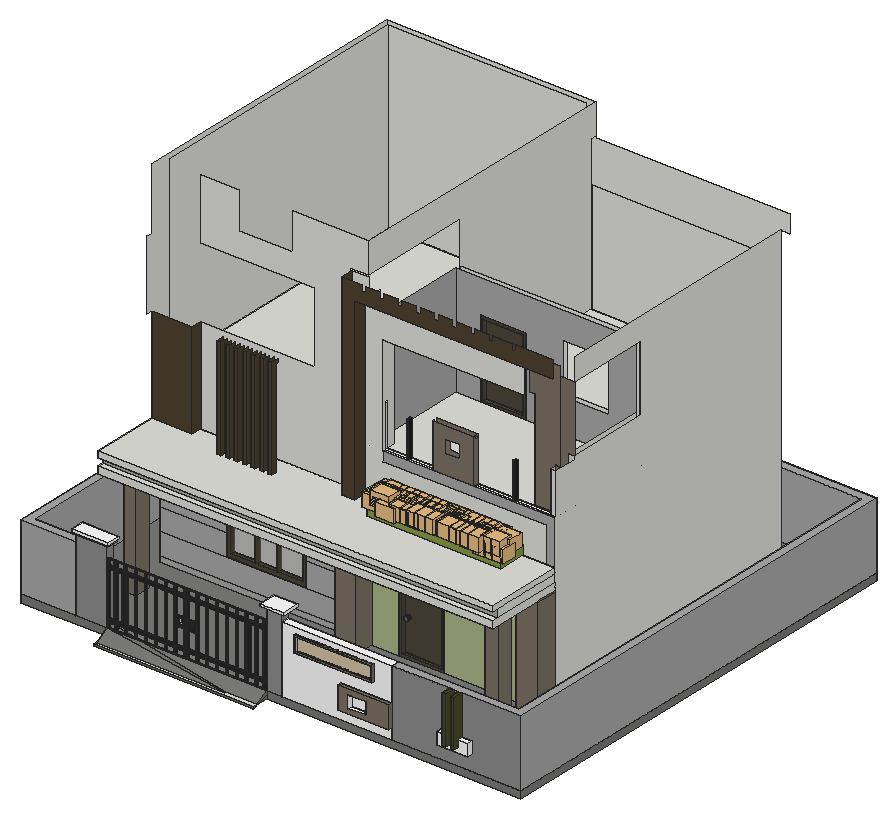
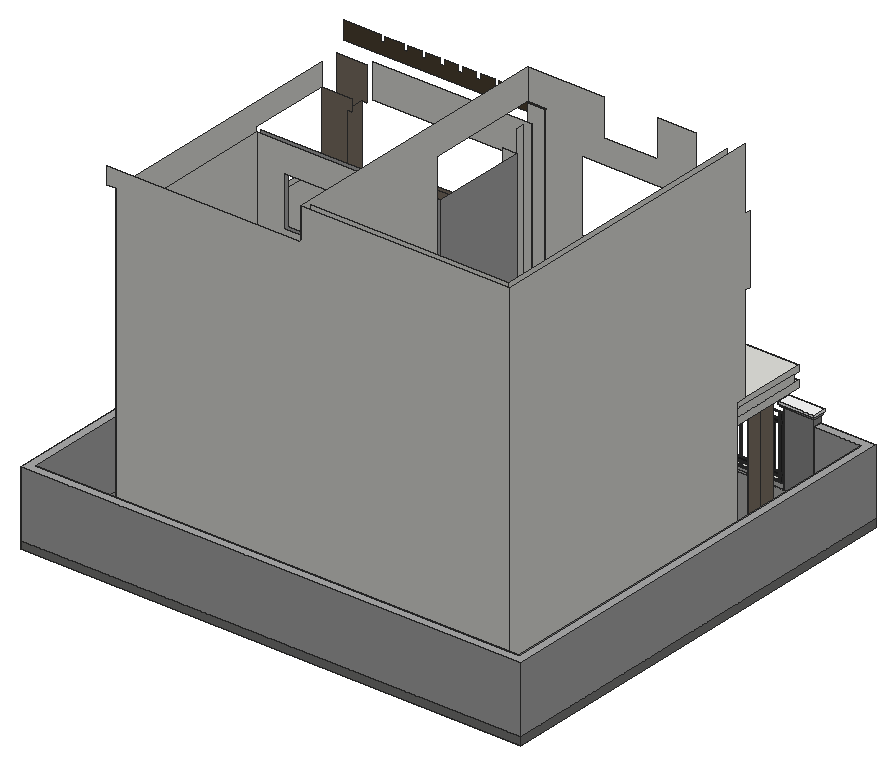
# SketchUp Ruby script. Lengths in inches.
U = 1.inch
M = Sketchup.active_model
def pt(a) = Geom::Point3d.new(a.map { |v| v * U })
def face(e, loops, mat)
  f = e.add_face(loops[0].map { |a| pt(a) })
  loops[1..].each { |l| e.add_face(l.map { |a| pt(a) }).erase! }
  f.material = f.back_material = mat if mat
  f
end
# faces: each face lists its corners as indices into pts; further lists are holes
def faces(e, pts, list, mat = nil) = list.each { |f| face(e, (f[0].is_a?(Array) ? f : [f]).map { |l| l.map { |i| pts[i] } }, mat) }
# xy, xz, yz: faces in a plane at the given z, y or x. An outline is a flat list of corners, or four numbers for a rectangle; further outlines are holes
def ring(l) = l.size == 4 ? [[l[0], l[1]], [l[2], l[1]], [l[2], l[3]], [l[0], l[3]]] : l.each_slice(2).to_a
def flat(e, list, mat, &to3) = list.each { |f| face(e, (f[0].is_a?(Array) ? f : [f]).map { |l| ring(l).map { |u, v| to3.(u, v) } }, mat) }
def xy(e, z, list, mat = nil) = flat(e, list, mat) { |x, y| [x, y, z] }
def xz(e, y, list, mat = nil) = flat(e, list, mat) { |x, z| [x, y, z] }
def yz(e, x, list, mat = nil) = flat(e, list, mat) { |y, z| [x, y, z] }
def lines(e, pts, list) = list.each { |a, b| e.add_line(pt(pts[a]), pt(pts[b])) }
# prism: a flat outline (further loops are holes) pulled along v
def prism(e, loops, v, mat = nil)
  f = face(e, loops, mat); d = Geom::Vector3d.new(v.map { |x| x * U })
  f.pushpull(f.normal.samedirection?(d) ? d.length : -d.length)
end
def box(e, o, s, mat = nil) = prism(e, [[o, [o[0] + s[0], o[1], o[2]], [o[0] + s[0], o[1] + s[1], o[2]], [o[0], o[1] + s[1], o[2]]]], [0, 0, s[2]], mat)
def at(x, y, z, deg = 0) = Geom::Transformation.translation(pt([x, y, z])) * Geom::Transformation.rotation(ORIGIN, Z_AXIS, deg.degrees)
def axes(o, x, y, z) = Geom::Transformation.new([*x, 0, *y, 0, *z, 0, *pt(o).to_a, 1])
def part(name) = M.definitions.add(name)
# library, detail: a bought-in or finely detailed component or shape, given as its bounding box
def library(name, o, s) = part(name).tap { |d| box(d.entities, o, s) }
def detail(e, o, s) = box(e.add_group.entities, o, s)
def put(e, d, t, mat = nil) = e.add_instance(d, t).tap { |i| i.material = mat if mat }
def group(e, t, mat = nil) = e.add_group.tap { |g| g.transformation = t; g.material = mat if mat }.entities
root = M.entities
M.materials.add("Calibrachoa hybrid Superbells  Cherry Blossom").color = [57, 76, 25]
M.materials.add("[Color B08]").color = [76, 71, 58]
M.materials.add("[Color C08]").color = [78, 67, 50]
M.materials.add("[Color D08]").color = [73, 76, 41]
M.materials.add("[Color M00]").color = [255, 255, 255]
M.materials.add("[Color M03]").color = [170, 170, 170]
M.materials.add("[Color M04]").color = [142, 142, 142]
M.materials.add("[Color M08]").color = [30, 30, 30]
M.materials.add("[Encaustic Tile Circular 01]").color = [123, 123, 122]
M.materials.add("[Grass Light Green]").color = [138, 158, 69]
M.materials.add("[Metal Corrugated Shiny]").color = [38, 38, 38]
M.materials.add("[Metal Seamed]").color = [87, 119, 115]
M.materials.add("[Metal Silver]").color = [234, 233, 238]
M.materials.add("[Square Glass Tile 04]").color = [171, 181, 136]
M.materials.add("[Stone Flagstone Ashlar]1").color = [126, 116, 102]
M.materials.add("[Tile Various Tan]").color = [214, 196, 169]
M.materials.add("[Translucent Glass Gray]").color = [128, 128, 128]
M.materials["[Translucent Glass Gray]"].alpha = 0.5
c1 = part("Group\#3")
xy(c1.entities,0,[[0,0,48,3.875]],"[Color B08]")
xy(c1.entities,2.57,[[2.57,0,45.43,3.875]],"[Color B08]")
xy(c1.entities,81.43,[[2.57,0,45.43,3.875]],"[Color B08]")
xy(c1.entities,84,[[0,0,48,3.875]],"[Color B08]")
xz(c1.entities,0,[[[0,0,48,84],[2.57,2.57,45.43,81.43]]],"[Color B08]")
xz(c1.entities,0.1875,[[6.99,35.83,7.61,35.84,8.2,36.01,8.73,36.33,9.17,36.77,9.47,37.3125,9.62,37.91,9.61,38.53,9.4375,39.13,9.12,39.66,8.67,40.09,8.13,40.39,7.53,40.54,6.91,40.53,6.3125,40.36,5.78,40.04,5.35,39.6,5.05,39.06,4.9,38.46,4.91,37.84,5.08,37.24,5.4,36.71,5.84,36.28,6.39,35.98]],"[Metal Seamed]")
xz(c1.entities,3.875,[[[0,0,48,84],[2.57,2.57,45.43,81.43]],[[2.57,2.57,45.43,81.43],[6.99,35.83,6.39,35.98,5.84,36.28,5.4,36.71,5.08,37.24,4.91,37.84,4.9,38.46,5.05,39.06,5.35,39.6,5.78,40.04,6.3125,40.36,6.91,40.53,7.53,40.54,8.13,40.39,8.67,40.09,9.12,39.66,9.4375,39.13,9.61,38.53,9.62,37.91,9.47,37.3125,9.17,36.77,8.73,36.33,8.2,36.01,7.61,35.84]]],"[Color B08]")
xz(c1.entities,3.875,[[6.99,35.83,6.39,35.98,5.84,36.28,5.4,36.71,5.08,37.24,4.91,37.84,4.9,38.46,5.05,39.06,5.35,39.6,5.78,40.04,6.3125,40.36,6.91,40.53,7.53,40.54,8.13,40.39,8.67,40.09,9.12,39.66,9.4375,39.13,9.61,38.53,9.62,37.91,9.47,37.3125,9.17,36.77,8.73,36.33,8.2,36.01,7.61,35.84]],"[Metal Seamed]")
yz(c1.entities,0,[[0,0,3.875,84]],"[Color B08]")
yz(c1.entities,2.57,[[0,2.57,3.875,81.43]],"[Color B08]")
yz(c1.entities,45.43,[[0,2.57,3.875,81.43]],"[Color B08]")
yz(c1.entities,48,[[0,0,3.875,84]],"[Color B08]")
p = [[6.39,3.875,35.98],[6.99,3.875,35.83],[6.99,0.1875,35.83],[6.39,0.1875,35.98],[7.61,3.875,35.84],[7.61,0.1875,35.84],
  [8.2,3.875,36.01],[8.2,0.1875,36.01],[5.84,3.875,36.28],[5.84,0.1875,36.28],[8.73,3.875,36.33],[8.73,0.1875,36.33],
  [5.4,3.875,36.71],[5.4,0.1875,36.71],[9.17,3.875,36.77],[9.17,0.1875,36.77],[5.08,3.875,37.24],[5.08,0.1875,37.24],
  [9.47,3.875,37.3125],[9.47,0.1875,37.3125],[4.91,3.875,37.84],[4.91,0.1875,37.84],[9.62,3.875,37.91],[9.62,0.1875,37.91],
  [4.9,3.875,38.46],[4.9,0.1875,38.46],[9.61,3.875,38.53],[9.61,0.1875,38.53],[5.05,3.875,39.06],[5.05,0.1875,39.06],
  [9.4375,3.875,39.13],[9.4375,0.1875,39.13],[5.35,3.875,39.6],[5.35,0.1875,39.6],[9.12,3.875,39.66],[9.12,0.1875,39.66],
  [5.78,3.875,40.04],[5.78,0.1875,40.04],[8.67,3.875,40.09],[8.67,0.1875,40.09],[6.3125,3.875,40.36],[6.3125,0.1875,40.36],
  [8.13,3.875,40.39],[8.13,0.1875,40.39],[6.91,3.875,40.53],[6.91,0.1875,40.53],[7.53,3.875,40.54],[7.53,0.1875,40.54]]
faces(c1.entities,p,[[0,1,2,3],[1,4,5,2],[4,6,7,5],[8,0,3,9],[6,10,11,7],[12,8,9,13],[10,14,15,11],[16,12,13,17],
  [14,18,19,15],[20,16,17,21],[18,22,23,19],[24,20,21,25],[22,26,27,23],[28,24,25,29],[26,30,31,27],[32,28,29,33],
  [30,34,35,31],[36,32,33,37],[34,38,39,35],[40,36,37,41],[38,42,43,39],[44,40,41,45],[42,46,47,43],[46,44,45,47]],"[Metal Seamed]")
c2 = part("Component\#24")
prism(c2.entities,[[[0,1.89,1.72],[0,1.6875,1.91],[0,1.44,2.04],[0,1.18,2.11],[0,0.9,2.11],[0,0.63,2.03],[0,0.39,1.89],[0,0.2,1.6875],[0,0.07,1.44],[0,0,1.18],[0,0,0.9],[0,0.08,0.63],[0,0.22,0.39],[0,0.42,0.2],[0,0.67,0.07],[0,0.9375,0],[0,1.21,0],[0,1.48,0.08],[0,1.72,0.22],[0,1.91,0.42],[0,2.04,0.67],[0,2.11,0.9375],[0,2.11,1.21],[0,2.03,1.48]]],[-0.625,0,0])
c3 = part("Gate cross rail")
box(c3.entities,[0,0,0],[3,48,2])
c4 = part("Gate edge rail")
box(c4.entities,[0,0.5625,0],[48,0.625,0.625])
c5 = part("Gate picket")
box(c5.entities,[0,0,0],[63,1.1875,0.625])
c6 = part("Gate cross rail \#1")
box(c6.entities,[0,0,0],[3,45,2])
c7 = part("Component\#23")
xy(c7.entities,0,[[0,0,11.01,4.67]])
c8 = part("Gate panel")
put(c8.entities,c3,at(54.625,0,0),"[Metal Corrugated Shiny]")
put(c8.entities,c4,axes([0.625,0,1.96],[0,1,0],[0,0,-1],[-1,0,0]),"[Metal Corrugated Shiny]")
put(c8.entities,c5,at(0.625,46.8125,0.78),"[Metal Corrugated Shiny]")
put(c8.entities,c3,at(6.625,0,0),"[Metal Corrugated Shiny]")
put(c8.entities,c5,at(0.625,10.8125,0.78),"[Metal Corrugated Shiny]")
put(c8.entities,c5,at(0.625,4.8125,0.78),"[Metal Corrugated Shiny]")
put(c8.entities,c4,axes([64.25,0,1.96],[0,1,0],[0,0,-1],[-1,0,0]),"[Metal Corrugated Shiny]")
put(c8.entities,c5,at(0.625,34.8125,0.78),"[Metal Corrugated Shiny]")
put(c8.entities,c5,at(0.625,28.8125,0.78),"[Metal Corrugated Shiny]")
put(c8.entities,c5,at(0.625,40.8125,0.78),"[Metal Corrugated Shiny]")
put(c8.entities,c6,at(9.625,12,0,-90),"[Metal Corrugated Shiny]")
put(c8.entities,c5,at(0.625,22.8125,0.78),"[Metal Corrugated Shiny]")
put(c8.entities,c5,at(0.625,0,0.78),"[Metal Corrugated Shiny]")
put(c8.entities,c5,at(0.625,16.8125,0.78),"[Metal Corrugated Shiny]")
put(c8.entities,c7,axes([26.47,42,1.4],[1,0,0],[0,1.14286,0],[0,0,1]),"[Metal Corrugated Shiny]")
c9 = part("Component\#25")
box(c9.entities,[-0.625,0,0],[0.625,0.9375,5.875])
c10 = part("Metal gate leaf")
put(c10.entities,c2,at(0.625,39.09,32.62),"[Metal Silver]")
put(c10.entities,c8,axes([2.03,0,0],[0,0,1],[0,0.875,0],[-1,0,0]))
put(c10.entities,c9,at(0.625,38.15,29.71),"[Metal Silver]")
c11 = part("Group\#2")
xy(c11.entities,0,[[0,0,90.375,3.1875]],"[Color B08]")
xy(c11.entities,4.18,[[4.18,0,31.5,3.1875],[31.5,0,33.18,3.1875],[33.18,0,56.375,3.1875],[56.375,0,58.06,3.1875],[58.06,0,86.19,3.1875]],"[Color B08]")
xy(c11.entities,71.26,[[4.18,0,31.5,3.1875],[33.18,0,56.375,3.1875],[58.06,0,86.19,3.1875]],"[Color B08]")
xy(c11.entities,75.4375,[[0,0,90.375,3.1875]],"[Color B08]")
xz(c11.entities,0,[[[0,0,90.375,75.4375],[4.18,4.18,4.18,71.26,31.5,71.26,31.5,4.18,33.18,4.18,33.18,71.26,56.375,71.26,56.375,4.18,58.06,4.18,58.06,71.26,86.19,71.26,86.19,4.18]]],"[Color B08]")
xz(c11.entities,3.1875,[[[0,0,90.375,75.4375],[4.18,4.18,86.19,4.18,86.19,71.26,58.06,71.26,58.06,4.18,56.375,4.18,56.375,71.26,33.18,71.26,33.18,4.18,31.5,4.18,31.5,71.26,4.18,71.26]]],"[Color B08]")
xz(c11.entities,3.1875,[[4.18,4.18,31.5,71.26],[33.18,4.18,56.375,71.26],[58.06,4.18,86.19,71.26]],"[Translucent Glass Gray]")
yz(c11.entities,0,[[0,0,3.1875,75.4375]],"[Color B08]")
yz(c11.entities,4.18,[[0,4.18,3.1875,71.26]],"[Color B08]")
yz(c11.entities,31.5,[[0,4.18,3.1875,71.26]],"[Color B08]")
yz(c11.entities,33.18,[[0,4.18,3.1875,71.26]],"[Color B08]")
yz(c11.entities,56.375,[[0,4.18,3.1875,71.26]],"[Color B08]")
yz(c11.entities,58.06,[[0,4.18,3.1875,71.26]],"[Color B08]")
yz(c11.entities,86.19,[[0,4.18,3.1875,71.26]],"[Color B08]")
yz(c11.entities,90.375,[[0,0,3.1875,75.4375]],"[Color B08]")
c12 = library("Calibrachoa hybrid Superbells  Cherry Blossom",[-6.55,-6.53,-1.33],[13.33,12.4,6.49])
xy(root,0,[[93.08,0,93.08,17,0,17,0,497,540,497,540,17,266,17,266,0]])
xy(root,8,[[460.82,67.49,475.94,84.3],[64.2,75.94,77.33,93.13],[264.14,111.75,264.14,134,57,134,57,440,483,440,483,134,363.43,134,363.43,140,477,140,477,434,63,434,63,140,315.43,140,315.43,134,285.95,134,285.95,111.75],[458.76,111.75,483,134],[63,140,477,434]])
xy(root,8,[[0,17,0,497,540,497,540,17,401.28,17,401.28,26,531,26,531,488,9,488,9,26,60.33,26,60.33,17],[60.33,17,93.08,26],[266,17,281.92,26],[281.92,17,401.28,26]],"[Color M00]")
xy(root,8,[[[9,26,531,488],[264.14,111.75,264.14,134,57,134,57,440,483,440,483,111.75,458.76,111.75,458.76,134,363.43,134,363.43,140,315.43,140,315.43,134,285.95,134,285.95,111.75],[460.82,67.49,475.94,84.3],[64.2,75.94,77.33,93.13]]],"[Encaustic Tile Circular 01]")
xy(root,19.88,[[346.36,12.625,401.28,17]],"[Stone Flagstone Ashlar]1")
xy(root,24.75,[[453.96,11.375,487.77,17]],"[Color M00]")
xy(root,25.0625,[[357.39,12.625,376.08,17]],"[Color M00]")
xy(root,28.93,[[463.45,7,467.76,11.375],[472.72,7,476.43,11.375]],"[Color D08]")
xy(root,37.25,[[453.96,11.375,463.45,17],[463.45,11.375,467.76,17],[467.76,11.375,472.72,17],[472.72,11.375,476.43,17],[476.43,11.375,487.77,17]],"[Color M00]")
xy(root,38.5625,[[357.39,12.625,376.08,17]],"[Color M00]")
xy(root,38.82,[[129.67,134,215.11,140]])
xy(root,43.8,[[346.36,12.625,401.28,17]],"[Stone Flagstone Ashlar]1")
xy(root,57.3125,[[297.52,14.5625,381.4,17]],"[Stone Flagstone Ashlar]1")
xy(root,58.67,[[298.88,14.5625,380.04,17]],"[Tile Various Tan]")
xy(root,72.89,[[298.88,14.5625,380.04,17]],"[Tile Various Tan]")
xy(root,74.25,[[297.52,14.5625,381.4,17]],"[Stone Flagstone Ashlar]1")
xy(root,80,[[463.45,7,467.76,17],[472.72,7,476.43,17]],"[Color D08]")
xy(root,80,[[281.92,17,401.28,26]],"[Color M00]")
xy(root,80,[[0,17,60.33,17,60.33,26,9,26,9,488,531,488,531,26,401.28,26,401.28,17,540,17,540,497,0,497]],"[Color M03]")
xy(root,88.0625,[[60.33,17,93.08,26],[266,17,281.92,26]],"[Color M00]")
xy(root,88.0625,[[[58.96,15.875,95.7,27.25],[60.33,17,93.08,26]],[[265.31,15.9375,283.8,28],[266,17,281.92,26]]],"[Color M04]")
xy(root,90.3125,[[[262.18,12.875,287.48,31.75],[265.31,15.9375,283.8,28]],[[57.77,13.75,97.39,28.5],[58.96,15.875,95.7,27.25]],[58.96,15.875,95.7,27.25],[265.31,15.9375,283.8,28]],"[Color M00]")
xy(root,92,[[315.43,134,363.43,140]])
xy(root,92.9375,[[262.18,12.875,287.48,31.75],[57.77,13.75,97.39,28.5]],"[Color M00]")
xy(root,113.63,[[129.67,134,215.11,140]])
xy(root,129.875,[[[57,50.5,57,134,264.14,134,264.14,111.75,285.95,111.75,285.95,134,458.76,134,458.76,111.75,483,111.75,483,50.5],[460.82,67.49,475.94,84.3]],[264.14,111.75,285.95,134],[458.76,111.75,483,134]])
xy(root,130.3125,[[64.2,75.94,77.33,93.13]])
xy(root,137.125,[[57,50.5,483,57.1875],[57,57.1875,483,134]])
xy(root,145.625,[[57,50.5,483,57.1875],[57,57.1875,483,134]])
xy(root,150.49,[[138.22,109.625,142.66,113.92]],"[Color M03]")
xy(root,152,[[[57,50.5,483,50.5,483,134,448.625,134,448.625,104.5625,303.4375,104.5625,303.4375,134,278.5625,134,278.5625,119.875,264.5625,119.875,264.5625,134,100.7,134,100.7,122.5625,57,122.5625],[193.35,109.625,197.78,113.92],[184.16,109.625,188.6,113.92],[174.97,109.625,179.41,113.92],[165.78,109.625,170.22,113.92],[156.6,109.625,161.03,113.92],[147.41,109.625,151.85,113.92]],[57,122.5625,100.7,134]])
xy(root,161.875,[[303.4375,104.5625,448.625,134]],"[Grass Light Green]")
xy(root,194,[[63,140,477,434]])
xy(root,200,[[351.41,134,395.45,140],[63,140,276.75,434],[282.75,140,297.76,148.25],[297.76,140,477,140,477,141.8125,455.38,141.8125,455.38,161.5,477,161.5,477,250.9375,358.04,250.9375,358.04,256.9375,310.04,256.9375,310.04,250.9375,282.75,250.9375,282.75,148.25,297.76,148.25],[455.38,141.8125,477,161.5],
  [282.75,256.9375,477,434]])
xy(root,200,[[297.76,134,351.41,136.1875],[395.45,134,483,136.1875],[297.76,136.1875,321.84,140],[324.02,136.1875,351.41,140],[395.45,136.1875,436.79,140],
  [439.16,136.1875,477,140]],"[Color M00]")
xy(root,200,[[321.84,136.1875,324.02,140],[436.79,136.1875,439.16,140]],"[Color M08]")
xz(root,0,[[93.08,-2.16,266,0]],"[Encaustic Tile Circular 01]")
xz(root,7,[[463.45,28.93,467.76,80],[472.72,28.93,476.43,80]],"[Color D08]")
xz(root,11.375,[[453.96,24.75,487.77,24.75,487.77,37.25,476.43,37.25,476.43,28.93,472.72,28.93,472.72,37.25,467.76,37.25,467.76,28.93,463.45,28.93,463.45,37.25,453.96,37.25]],"[Color M00]")
xz(root,11.375,[[463.45,28.93,467.76,37.25],[472.72,28.93,476.43,37.25]],"[Color M04]")
xz(root,12.625,[[[346.36,19.88,401.28,43.8],[357.39,25.0625,376.08,38.5625]]],"[Stone Flagstone Ashlar]1")
xz(root,12.875,[[262.18,90.3125,287.48,92.9375]],"[Color M00]")
xz(root,13.75,[[57.77,90.3125,97.39,92.9375]],"[Color M00]")
xz(root,14.5625,[[[297.52,57.3125,381.4,74.25],[298.88,58.67,380.04,72.89]]],"[Stone Flagstone Ashlar]1")
xz(root,15.875,[[58.96,88.0625,95.7,90.3125]],"[Color M04]")
xz(root,15.9375,[[265.31,88.0625,283.8,90.3125]],"[Color M04]")
xz(root,17,[[472.72,37.25,476.43,80]])
xz(root,17,[[[281.92,8,401.28,8,401.28,19.88,346.36,19.88,346.36,43.8,401.28,43.8,401.28,80,281.92,80],[297.52,57.3125,381.4,74.25]],[[346.36,19.88,401.28,43.8],[357.39,25.0625,376.08,38.5625]],[453.96,24.75,487.77,37.25],[357.39,25.0625,376.08,38.5625],[[297.52,57.3125,381.4,74.25],[298.88,58.67,380.04,72.89]]],"[Color M00]")
xz(root,17,[[0,8,60.33,80]],"[Color M03]")
xz(root,17,[[60.33,8,93.08,88.0625],[266,8,281.92,88.0625],[401.28,8,540,8,540,80,476.43,80,476.43,37.25,487.77,37.25,487.77,24.75,453.96,24.75,453.96,37.25,463.45,37.25,463.45,80,401.28,80],[463.45,37.25,467.76,80],[467.76,37.25,472.72,80]],"[Color M04]")
xz(root,17,[[0,0,93.08,8],[266,0,540,8]],"[Encaustic Tile Circular 01]")
xz(root,17,[[298.88,58.67,380.04,72.89]],"[Tile Various Tan]")
xz(root,26,[[9,8,60.33,80],[281.92,8,401.28,80],[401.28,8,531,80]],"[Color M03]")
xz(root,26,[[60.33,8,93.08,88.0625],[266,8,281.92,88.0625]],"[Color M04]")
xz(root,27.25,[[58.96,88.0625,95.7,90.3125]],"[Color M04]")
xz(root,28,[[265.31,88.0625,283.8,90.3125]],"[Color M04]")
xz(root,28.5,[[57.77,90.3125,97.39,92.9375]],"[Color M00]")
xz(root,31.75,[[262.18,90.3125,287.48,92.9375]],"[Color M00]")
xz(root,50.5,[[57,129.875,483,137.125],[57,145.625,483,152]])
xz(root,57.1875,[[57,137.125,483,145.625]],"[Color M03]")
xz(root,67.49,[[460.82,8,475.94,129.875]],"[Stone Flagstone Ashlar]1")
xz(root,75.94,[[64.2,8,77.33,130.3125]],"[Stone Flagstone Ashlar]1")
xz(root,84.3,[[460.82,8,475.94,129.875]])
xz(root,93.13,[[64.2,8,77.33,130.3125]],"[Stone Flagstone Ashlar]1")
xz(root,104.5625,[[303.4375,152,448.625,161.875]],"[Grass Light Green]")
xz(root,109.625,[[138.22,150.49,142.66,261.3],[147.41,152,151.85,261.3],[156.6,152,161.03,261.3],[165.78,152,170.22,261.3],[174.97,152,179.41,261.3],
  [184.16,152,188.6,261.3],[193.35,152,197.78,261.3]],"[Color C08]")
xz(root,111.75,[[264.14,8,285.95,129.875],[458.76,8,483,129.875]],"[Stone Flagstone Ashlar]1")
xz(root,113.92,[[138.22,150.49,142.66,257.55],[147.41,152,151.85,257.55],[156.6,152,161.03,257.55],[165.78,152,170.22,257.55],[174.97,152,179.41,257.55],
  [184.16,152,188.6,257.55],[193.35,152,197.78,257.55]],"[Color C08]")
xz(root,119.875,[[264.5625,152,278.5625,152,278.5625,344,492.4375,344,492.4375,362.625,452.77,362.625,452.77,356.93,447.96,356.93,447.96,362.625,427.83,362.625,427.83,356.93,423.02,356.93,423.02,362.625,408.27,362.625,408.27,356.93,403.46,356.93,403.46,362.625,388.71,362.625,388.71,356.93,383.89,356.93,383.89,362.625,369.14,362.625,369.14,356.93,364.33,356.93,364.33,362.625,349.58,362.625,349.58,356.93,344.77,356.93,344.77,362.625,330.02,362.625,330.02,356.93,325.21,356.93,325.21,362.625,310.46,362.625,310.46,356.93,305.64,356.93,305.64,362.625,290.89,362.625,290.89,356.93,286.08,356.93,286.08,362.625,264.5625,362.625]],"[Color C08]")
xz(root,122.5625,[[57,152,100.7,255.68]],"[Color C08]")
xz(root,134,[[458.76,8,483,129.875],[57,129.875,483,137.125],[57,137.125,483,145.625],[57,145.625,57,152,303.4375,152,303.4375,161.875,448.625,161.875,448.625,152,483,152,483,145.625],[100.7,152,264.5625,152,264.5625,362.625,261.625,362.625,261.625,364.625,282.75,364.625,282.75,397.5625,200.45,397.5625,200.45,358,142.38,358,142.38,397.5625,100.7,397.5625,100.7,331.68,224.8125,331.68,224.8125,255.68,100.7,255.68],
  [264.5625,152,278.5625,200],[278.5625,152,303.4375,152,303.4375,161.875,448.625,161.875,448.625,152,473.17,152,473.17,189.71,297.76,189.71,297.76,307.0625,450.07,307.0625,450.07,344,278.5625,344],[264.5625,200,278.5625,200,278.5625,344,282.75,344,282.75,362.625,264.5625,362.625]])
xz(root,134,[[57,8,264.14,8,264.14,13.79,215.11,13.79,129.67,13.85,57,13.85],[215.11,13.79,264.14,13.79,264.14,37.98,57,37.98,57,13.85,129.67,13.85],[57,37.98,264.14,37.98,264.14,64.04,215.11,64.04,215.11,38.82,129.67,38.82,129.67,61.54,57,61.54],[57,61.54,129.67,86.23],[215.11,64.04,264.14,88.6],
  [57,86.23,129.67,109.35],[215.11,88.6,264.14,109.35],[57,109.35,129.67,109.35,129.67,113.63,215.11,113.63,215.11,109.35,264.14,109.35,264.14,129.875,57,129.875],[473.17,152,483,152,483,200,297.76,200,297.76,189.71,473.17,189.71]],"[Color M03]")
xz(root,134,[[285.95,8,315.43,8,315.43,92,363.43,92,363.43,8,458.76,8,458.76,129.875,285.95,129.875]],"[Square Glass Tile 04]")
xz(root,134,[[[351.41,200,395.45,248],[364.68,220.77,380.63,235.41]]],"[Stone Flagstone Ashlar]1")
xz(root,136.1875,[[477,200,483,244.375]])
xz(root,136.1875,[[321.84,200,324.02,238.64],[436.79,200,439.16,238.64]],"[Color M08]")
xz(root,140,[[[63,8,63,152,477,152,477,8,363.43,8,363.43,92,315.43,92,315.43,8],[129.67,38.82,215.11,113.63]],[63,152,477,194],[63,194,477,200]])
xz(root,140,[[321.84,200,324.02,238.64],[436.79,200,439.16,238.64]],"[Color M08]")
xz(root,140,[[[351.41,200,395.45,248],[365.56,221.65,379.75,234.53]]],"[Stone Flagstone Ashlar]1")
xz(root,141.8125,[[455.38,200,477,200,477,246.375,483,246.375,483,344,450.07,344,450.07,307.0625,455.38,307.0625]],"[Stone Flagstone Ashlar]1")
xz(root,148.25,[[282.75,200,297.76,320]])
xz(root,161.5,[[455.38,200,455.38,307.0625,450.07,307.0625,450.07,320,483,320,483,248,477,248,477,200]],"[Stone Flagstone Ashlar]1")
xz(root,250.9375,[[[282.75,200,310.04,200,310.04,284,358.04,284,358.04,200,477,200,477,320,282.75,320],[398.45,236.42,448.01,291.17]]],"[Color M03]")
xz(root,256.9375,[[[282.75,200,282.75,320,477,320,477,200,358.04,200,358.04,284,310.04,284,310.04,200],[398.45,236.42,448.01,291.17]]])
xz(root,434,[[63,8,477,128],[63,128,477,152],[63,152,477,194],[63,194,215.91,200],[283.22,194,477,200],
  [63,200,276.75,397.5625],[282.75,200,283.22,320],[283.22,200,477,320]])
xz(root,440,[[57,8,57,397.5625,282.75,397.5625,282.75,362.625,492.4375,362.625,492.4375,344,483,344,483,8]])
xz(root,488,[[9,8,531,80]],"[Color M03]")
xz(root,497,[[0,8,540,80]],"[Color M03]")
xz(root,497,[[0,0,540,8]],"[Encaustic Tile Circular 01]")
yz(root,0,[[17,8,497,80]],"[Color M03]")
yz(root,0,[[17,0,497,8]],"[Encaustic Tile Circular 01]")
yz(root,9,[[26,8,488,80]],"[Color M03]")
yz(root,57,[[134,8,134,152,122.5625,152,122.5625,255.68,117.0625,255.68,117.0625,330.3,122.5625,330.3,122.5625,397.5625,440,397.5625,440,8],[50.5,129.875,134,137.125],[57.1875,137.125,134,145.625],[50.5,145.625,134,152]])
yz(root,57.77,[[13.75,90.3125,28.5,92.9375]],"[Color M00]")
yz(root,58.96,[[15.875,88.0625,27.25,90.3125]],"[Color M04]")
yz(root,60.33,[[17,8,26,80]],"[Color M00]")
yz(root,60.33,[[17,80,26,88.0625]],"[Color M04]")
yz(root,63,[[140,8,434,128],[140,128,434,152],[140,152,434,194],[140,194,434,200],[140,200,434,397.5625]])
yz(root,64.2,[[75.94,8,93.13,130.3125]],"[Stone Flagstone Ashlar]1")
yz(root,77.33,[[75.94,8,93.13,130.3125]],"[Stone Flagstone Ashlar]1")
yz(root,93.08,[[17,8,26,88.0625]],"[Color M04]")
yz(root,93.08,[[0,-2.16,3.61,0,17,8,17,0,0,0]],"[Encaustic Tile Circular 01]")
yz(root,95.7,[[15.875,88.0625,27.25,90.3125]],"[Color M04]")
yz(root,97.39,[[13.75,90.3125,28.5,92.9375]],"[Color M00]")
yz(root,100.7,[[122.5625,152,134,255.68]],"[Color C08]")
yz(root,129.67,[[134,38.82,140,113.63]])
yz(root,138.22,[[109.625,150.49,109.625,261.3,117.0625,261.3,117.0625,257.55,113.92,257.55,113.92,150.49]],"[Color C08]")
yz(root,142.66,[[109.625,150.49,113.92,150.49,113.92,257.55,117.0625,257.55,117.0625,261.3,109.625,261.3]],"[Color C08]")
yz(root,147.41,[[109.625,152,109.625,261.3,117.0625,261.3,117.0625,257.55,113.92,257.55,113.92,152]],"[Color C08]")
yz(root,151.85,[[109.625,152,113.92,152,113.92,257.55,117.0625,257.55,117.0625,261.3,109.625,261.3]],"[Color C08]")
yz(root,156.6,[[109.625,152,109.625,261.3,117.0625,261.3,117.0625,257.55,113.92,257.55,113.92,152]],"[Color C08]")
yz(root,161.03,[[109.625,152,113.92,152,113.92,257.55,117.0625,257.55,117.0625,261.3,109.625,261.3]],"[Color C08]")
yz(root,165.78,[[109.625,152,109.625,261.3,117.0625,261.3,117.0625,257.55,113.92,257.55,113.92,152]],"[Color C08]")
yz(root,170.22,[[109.625,152,113.92,152,113.92,257.55,117.0625,257.55,117.0625,261.3,109.625,261.3]],"[Color C08]")
yz(root,174.97,[[109.625,152,109.625,261.3,117.0625,261.3,117.0625,257.55,113.92,257.55,113.92,152]],"[Color C08]")
yz(root,179.41,[[109.625,152,113.92,152,113.92,257.55,117.0625,257.55,117.0625,261.3,109.625,261.3]],"[Color C08]")
yz(root,184.16,[[109.625,152,109.625,261.3,117.0625,261.3,117.0625,257.55,113.92,257.55,113.92,152]],"[Color C08]")
yz(root,188.6,[[109.625,152,113.92,152,113.92,257.55,117.0625,257.55,117.0625,261.3,109.625,261.3]],"[Color C08]")
yz(root,193.35,[[109.625,152,109.625,261.3,117.0625,261.3,117.0625,257.55,113.92,257.55,113.92,152]],"[Color C08]")
yz(root,197.78,[[109.625,152,113.92,152,113.92,257.55,117.0625,257.55,117.0625,261.3,109.625,261.3]],"[Color C08]")
yz(root,215.11,[[134,38.82,140,113.63]])
yz(root,262.18,[[12.875,90.3125,31.75,92.9375]],"[Color M00]")
yz(root,264.14,[[111.75,8,134,129.875]],"[Stone Flagstone Ashlar]1")
yz(root,264.5625,[[119.875,152,134,362.625]],"[Color C08]")
yz(root,265.31,[[15.9375,88.0625,28,90.3125]],"[Color M04]")
yz(root,266,[[17,8,26,88.0625]],"[Color M04]")
yz(root,266,[[0,-2.16,0,0,5.53,0,17,4.48,17,8,3.61,0],[0,-2.16,5.53,0,3.61,0],[5.53,0,17,0,17,4.48],[17,4.48,26,8,17,8]],"[Encaustic Tile Circular 01]")
yz(root,278.5625,[[119.875,152,134,344]],"[Color C08]")
yz(root,281.92,[[17,8,26,80]],"[Color M00]")
yz(root,281.92,[[17,80,26,88.0625]],"[Color M04]")
yz(root,282.75,[[256.9375,200,434,200,434,364.625,440,364.625,440,397.5625,134,397.5625,134,364.625,256.9375,364.625],[140,200,148.25,344]])
yz(root,282.75,[[148.25,200,250.9375,320]],"[Color M03]")
yz(root,283.8,[[15.9375,88.0625,28,90.3125]],"[Color M04]")
yz(root,285.95,[[111.75,8,134,129.875]],"[Stone Flagstone Ashlar]1")
yz(root,287.48,[[12.875,90.3125,31.75,92.9375]],"[Color M00]")
yz(root,297.52,[[14.5625,57.3125,17,74.25]],"[Stone Flagstone Ashlar]1")
yz(root,297.76,[[134,200,136.1875,200,136.1875,246.375,140,246.375,140,200,148.25,200,148.25,307.0625,134,307.0625],[[136.1875,200,140,244.375],[136.85,238.64,139.48,240.27],[137.5,230.29,139.18,231.72],[137.5,225.35,139.18,226.79],[137.5,220.41,139.18,221.85],[137.5,215.47,139.18,216.91],[137.5,210.54,139.18,211.97],[137.5,205.6,139.18,207.04]]])
yz(root,298.88,[[14.5625,58.67,17,72.89]],"[Tile Various Tan]")
yz(root,303.4375,[[104.5625,152,134,161.875]],"[Grass Light Green]")
yz(root,310.04,[[250.9375,200,256.9375,284]])
yz(root,315.43,[[134,8,140,92]])
yz(root,321.84,[[136.1875,200,140,238.64]],"[Color M08]")
yz(root,324.02,[[136.1875,200,140,238.64]],"[Color M08]")
yz(root,346.36,[[12.625,19.88,17,43.8]],"[Stone Flagstone Ashlar]1")
yz(root,351.41,[[[134,200,134,248,136.1875,248,136.1875,244.375,140,244.375,140,200],[137.5,230.29,139.18,231.72],[137.5,225.35,139.18,226.79],[137.5,220.41,139.18,221.85],[137.5,205.6,139.18,207.04]]],"[Stone Flagstone Ashlar]1")
yz(root,357.39,[[12.625,25.0625,17,38.5625]],"[Color M00]")
yz(root,358.04,[[250.9375,200,256.9375,284]])
yz(root,363.43,[[134,8,140,92]])
yz(root,376.08,[[12.625,25.0625,17,38.5625]],"[Color M00]")
yz(root,380.04,[[14.5625,58.67,17,72.89]],"[Tile Various Tan]")
yz(root,381.4,[[14.5625,57.3125,17,74.25]],"[Stone Flagstone Ashlar]1")
yz(root,395.45,[[[134,200,140,200,140,244.375,136.1875,244.375,136.1875,246.375,140,246.375,140,248,134,248],[137.57,230.3,139.26,231.73]]],"[Stone Flagstone Ashlar]1")
yz(root,401.28,[[17,8,26,80]],"[Color M00]")
yz(root,401.28,[[12.625,19.88,17,43.8]],"[Stone Flagstone Ashlar]1")
yz(root,436.79,[[136.1875,200,140,238.64]],"[Color M08]")
yz(root,439.16,[[136.1875,200,140,238.64]],"[Color M08]")
yz(root,448.625,[[104.5625,152,134,161.875]],"[Grass Light Green]")
yz(root,453.96,[[11.375,24.75,17,37.25]],"[Color M00]")
yz(root,455.38,[[141.8125,200,161.5,307.0625]],"[Stone Flagstone Ashlar]1")
yz(root,458.76,[[111.75,8,134,129.875]],"[Stone Flagstone Ashlar]1")
yz(root,460.82,[[67.49,8,84.3,129.875]],"[Stone Flagstone Ashlar]1")
yz(root,463.45,[[7,28.93,7,80,17,80,17,37.25,11.375,37.25,11.375,28.93]],"[Color D08]")
yz(root,467.76,[[7,28.93,11.375,28.93,11.375,37.25,17,37.25,17,80,7,80]],"[Color D08]")
yz(root,472.72,[[7,28.93,7,80,17,80,17,37.25,11.375,37.25,11.375,28.93]],"[Color D08]")
yz(root,475.94,[[67.49,8,84.3,129.875]],"[Stone Flagstone Ashlar]1")
yz(root,476.43,[[7,28.93,11.375,28.93,11.375,37.25,17,37.25,17,80,7,80]],"[Color D08]")
yz(root,477,[[140,8,434,128],[140,128,434,194],[137.57,198.8,139.26,200],[[136.1875,200,136.1875,244.375,141.8125,244.375,141.8125,200,139.26,200,139.26,200.23,137.57,200.23,137.57,200],[137.57,230.3,139.26,231.73],[137.57,225.05,139.26,226.48],[137.57,219.8,139.26,221.23],[137.57,214.55,139.26,215.98],[137.57,209.3,139.26,210.73],[137.57,204.05,139.26,205.48]],[137.57,200,139.26,200.23],
  [161.5,200,250.9375,248],[256.9375,200,434,320]])
yz(root,483,[[134,8,440,8,440,344,161.5,344,161.5,320,250.9375,320,250.9375,248,161.5,248,161.5,244.375,136.1875,244.375,136.1875,200,134,200],[50.5,129.875,134,137.125],[57.1875,137.125,134,145.625],[50.5,145.625,134,152]])
yz(root,483,[[111.75,8,134,128],[111.75,128,134,129.875]],"[Stone Flagstone Ashlar]1")
yz(root,487.77,[[11.375,24.75,17,37.25]],"[Color M00]")
yz(root,531,[[26,8,488,80]],"[Color M03]")
yz(root,540,[[17,8,497,80]],"[Color M03]")
yz(root,540,[[17,0,497,8]],"[Encaustic Tile Circular 01]")
p = [[93.08,0,-2.16],[266,0,-2.16],[93.08,17,8],[93.08,3.61,0],[93.08,26,8],[266,26,8],
  [266,5.53,0],[266,17,4.48],[477,250.9375,200],[477,256.9375,200],[282.75,134,200],[282.75,140,200],
  [483,250.9375,200],[477,161.5,200],[483,161.5,200],[483,141.8125,200],[477,141.8125,200],[483,148.25,200],
  [477,148.25,200],[477,140,230.29],[477,140,200],[477,136.85,238.64],[477,136.85,200],[711.63,-150.32,97.32],
  [711.63,-150.32,99.45]]
faces(root,p,[[0,1,2,3],[4,2,1],[5,4,1,6,7]],"[Encaustic Tile Circular 01]")
lines(root,p,[[8,9],[10,11],[12,8],[13,14],[15,16],[17,18],[19,20],[21,22],[23,24]])
put(root,c1,at(315.43,134,8))
g1 = group(root,at(93.08,17,8))
put(g1,c10,axes([170.6,0,0],[0,1,0],[-2.031,0,0],[0,0,1.06]))
put(g1,c10,axes([0,0,68.11],[0,1,0],[2.031,0,0],[0,0,-1.06]))
put(root,c11,axes([129.61,134,38.82],[0.946,0,0],[0,1.3442,0],[0,0,0.99171]))
put(root,c12,axes([356.74,138.48,159.07],[1.5,0,0],[0,1.24,0],[0,0,2.18]))
put(root,c12,axes([328.88,114.15,159.17],[1.5,0,0],[0,1.24,0],[0,0,2.18]))
put(root,c12,axes([428.49,112.65,159.83],[1.5,0,0],[0,1.24,0],[0,0,2.18]))
put(root,c12,axes([440.74,112.65,159.83],[1.5,0,0],[0,1.24,0],[0,0,2.18]))
put(root,c12,axes([370.18,134.16,160.21],[1.5,0,0],[0,1.24,0],[0,0,2.18]))
put(root,c12,axes([383.62,129.83,161.35],[1.5,0,0],[0,1.24,0],[0,0,2.18]))
put(root,c12,axes([419.7,112.65,162.45],[1.5,0,0],[0,1.24,0],[0,0,2.18]))
put(root,c12,axes([397.06,125.51,162.49],[1.5,0,0],[0,1.24,0],[0,0,2.18]))
put(root,c12,axes([309.66,127.82,162.99],[1.5,0,0],[0,1.24,0],[0,0,2.18]))
put(root,c12,axes([309.66,121.45,162.99],[1.5,0,0],[0,1.24,0],[0,0,2.18]))
put(root,c12,axes([309.66,115.39,162.99],[1.5,0,0],[0,1.24,0],[0,0,2.18]))
put(root,c12,axes([309.66,111.32,162.99],[1.5,0,0],[0,1.24,0],[0,0,2.18]))
put(root,c12,axes([382,120.6875,163.02],[1.5,0,0],[0,1.24,0],[0,0,2.18]))
put(root,c12,axes([382,111.4375,163.02],[1.5,0,0],[0,1.24,0],[0,0,2.18]))
put(root,c12,axes([328.58,104.95,163.21],[1.5,0,0],[0,1.24,0],[0,0,2.18]))
put(root,c12,axes([410.49,121.18,163.63],[1.5,0,0],[0,1.24,0],[0,0,2.18]))
put(root,c12,axes([423.93,116.85,164.77],[1.5,0,0],[0,1.24,0],[0,0,2.18]))
put(root,c12,axes([411.8,112.65,164.77],[1.5,0,0],[0,1.24,0],[0,0,2.18]))
put(root,c12,axes([421.8,112.65,164.77],[1.5,0,0],[0,1.24,0],[0,0,2.18]))
put(root,c12,axes([399.94,112.65,164.77],[1.5,0,0],[0,1.24,0],[0,0,2.18]))
put(root,c12,axes([389.4,118,164.77],[1.5,0,0],[0,1.24,0],[0,0,2.18]))
put(root,c12,axes([389.4,109.93,164.77],[1.5,0,0],[0,1.24,0],[0,0,2.18]))
put(root,c12,axes([380.5625,121.89,164.77],[1.5,0,0],[0,1.24,0],[0,0,2.18]))
put(root,c12,axes([366.81,118.67,164.77],[1.5,0,0],[0,1.24,0],[0,0,2.18]))
put(root,c12,axes([354.43,118.67,164.77],[1.5,0,0],[0,1.24,0],[0,0,2.18]))
put(root,c12,axes([341.5,118.67,164.77],[1.5,0,0],[0,1.24,0],[0,0,2.18]))
put(root,c12,axes([334.81,118.67,164.77],[1.5,0,0],[0,1.24,0],[0,0,2.18]))
put(root,c12,axes([324.56,118.67,164.77],[1.5,0,0],[0,1.24,0],[0,0,2.18]))
put(root,c12,axes([317.43,118.67,164.77],[1.5,0,0],[0,1.24,0],[0,0,2.18]))
put(root,c12,axes([342.46,106.95,164.77],[1.5,0,0],[0,1.24,0],[0,0,2.18]))
put(root,c12,axes([353.9,106.95,164.77],[1.5,0,0],[0,1.24,0],[0,0,2.18]))
put(root,c12,axes([316.72,125.875,164.77],[1.5,0,0],[0,1.24,0],[0,0,2.18]))
put(root,c12,axes([330.91,125.875,164.77],[1.5,0,0],[0,1.24,0],[0,0,2.18]))
put(root,c12,axes([344.6,125.875,164.77],[1.5,0,0],[0,1.24,0],[0,0,2.18]))
put(root,c12,axes([360.47,125.875,164.77],[1.5,0,0],[0,1.24,0],[0,0,2.18]))
put(root,c12,axes([372.85,125.875,164.77],[1.5,0,0],[0,1.24,0],[0,0,2.18]))
put(root,c12,axes([385.1,125.875,164.77],[1.5,0,0],[0,1.24,0],[0,0,2.18]))
put(root,c12,axes([400.54,125.875,164.77],[1.5,0,0],[0,1.24,0],[0,0,2.18]))
put(root,c12,axes([414.97,125.875,164.77],[1.5,0,0],[0,1.24,0],[0,0,2.18]))
put(root,c12,axes([427.41,125.875,164.77],[1.5,0,0],[0,1.24,0],[0,0,2.18]))
put(root,c12,axes([427.92,112.65,164.83],[1.5,0,0],[0,1.24,0],[0,0,2.18]))
put(root,c12,axes([440.36,122.625,165.23],[1.5,0,0],[0,1.24,0],[0,0,2.18]))
put(root,c12,axes([437.37,112.53,165.91],[1.5,0,0],[0,1.24,0],[0,0,2.18]))
put(root,c12,axes([361.12,106.59,166.16],[1.5,0,0],[0,1.24,0],[0,0,2.18]))
put(root,c12,axes([369.68,106.59,166.16],[1.5,0,0],[0,1.24,0],[0,0,2.18]))
put(root,c12,axes([394.3,106.59,166.16],[1.5,0,0],[0,1.24,0],[0,0,2.18]))
put(root,c12,axes([407.37,106.59,166.16],[1.5,0,0],[0,1.24,0],[0,0,2.18]))
put(root,c12,axes([419.55,106.59,166.16],[1.5,0,0],[0,1.24,0],[0,0,2.18]))
put(root,c12,axes([318.16,111.32,167.93],[1.5,0,0],[0,1.24,0],[0,0,2.18]))
put(root,c1,at(310.04,250.9375,200))
